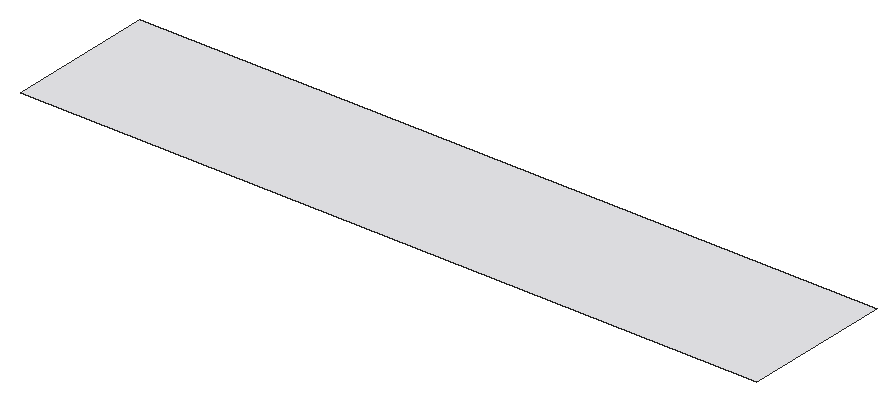
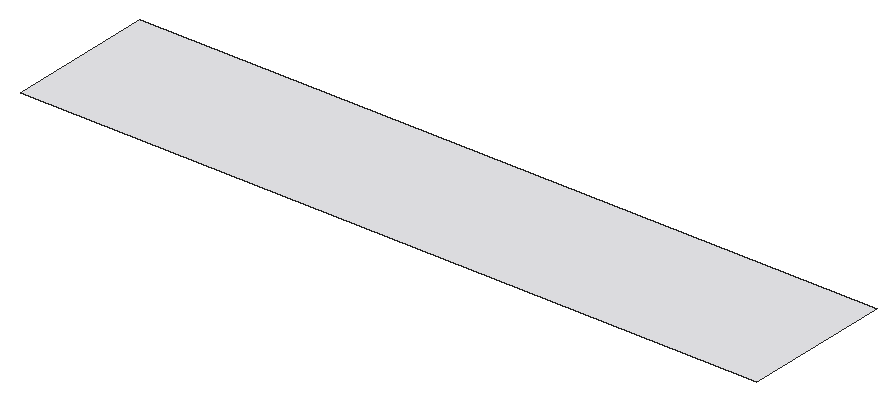
# SketchUp Ruby script. Lengths in inches.
U = 1.inch
M = Sketchup.active_model
def pt(a) = Geom::Point3d.new(a.map { |v| v * U })
def face(e, loops, mat)
  f = e.add_face(loops[0].map { |a| pt(a) })
  loops[1..].each { |l| e.add_face(l.map { |a| pt(a) }).erase! }
  f.material = f.back_material = mat if mat
  f
end
# faces: each face lists its corners as indices into pts; further lists are holes
def faces(e, pts, list, mat = nil) = list.each { |f| face(e, (f[0].is_a?(Array) ? f : [f]).map { |l| l.map { |i| pts[i] } }, mat) }
# xy, xz, yz: faces in a plane at the given z, y or x. An outline is a flat list of corners, or four numbers for a rectangle; further outlines are holes
def ring(l) = l.size == 4 ? [[l[0], l[1]], [l[2], l[1]], [l[2], l[3]], [l[0], l[3]]] : l.each_slice(2).to_a
def flat(e, list, mat, &to3) = list.each { |f| face(e, (f[0].is_a?(Array) ? f : [f]).map { |l| ring(l).map { |u, v| to3.(u, v) } }, mat) }
def xy(e, z, list, mat = nil) = flat(e, list, mat) { |x, y| [x, y, z] }
def xz(e, y, list, mat = nil) = flat(e, list, mat) { |x, z| [x, y, z] }
def yz(e, x, list, mat = nil) = flat(e, list, mat) { |y, z| [x, y, z] }
def lines(e, pts, list) = list.each { |a, b| e.add_line(pt(pts[a]), pt(pts[b])) }
# prism: a flat outline (further loops are holes) pulled along v
def prism(e, loops, v, mat = nil)
  f = face(e, loops, mat); d = Geom::Vector3d.new(v.map { |x| x * U })
  f.pushpull(f.normal.samedirection?(d) ? d.length : -d.length)
end
def box(e, o, s, mat = nil) = prism(e, [[o, [o[0] + s[0], o[1], o[2]], [o[0] + s[0], o[1] + s[1], o[2]], [o[0], o[1] + s[1], o[2]]]], [0, 0, s[2]], mat)
def at(x, y, z, deg = 0) = Geom::Transformation.translation(pt([x, y, z])) * Geom::Transformation.rotation(ORIGIN, Z_AXIS, deg.degrees)
def axes(o, x, y, z) = Geom::Transformation.new([*x, 0, *y, 0, *z, 0, *pt(o).to_a, 1])
def part(name) = M.definitions.add(name)
# library, detail: a bought-in or finely detailed component or shape, given as its bounding box
def library(name, o, s) = part(name).tap { |d| box(d.entities, o, s) }
def detail(e, o, s) = box(e.add_group.entities, o, s)
def put(e, d, t, mat = nil) = e.add_instance(d, t).tap { |i| i.material = mat if mat }
def group(e, t, mat = nil) = e.add_group.tap { |g| g.transformation = t; g.material = mat if mat }.entities
root = M.entities
M.materials.add("[Blinds Vertical Pattern]1").color = [239, 239, 242]
xy(root,37.78,[[213.78,96.24,286.85,111]],"[Blinds Vertical Pattern]1")
